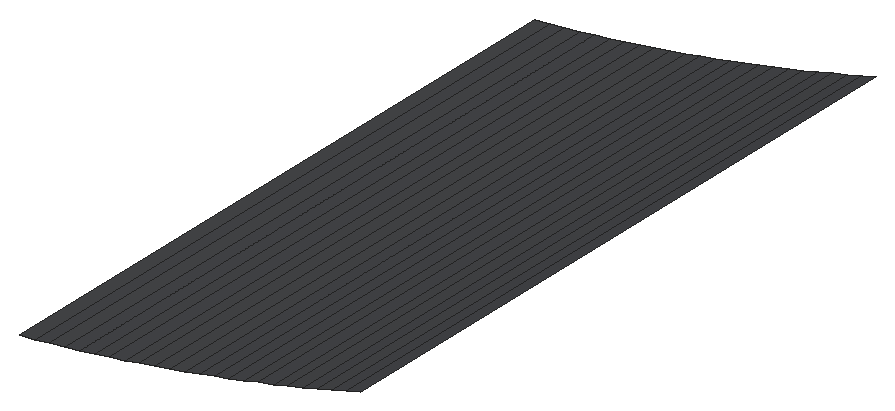
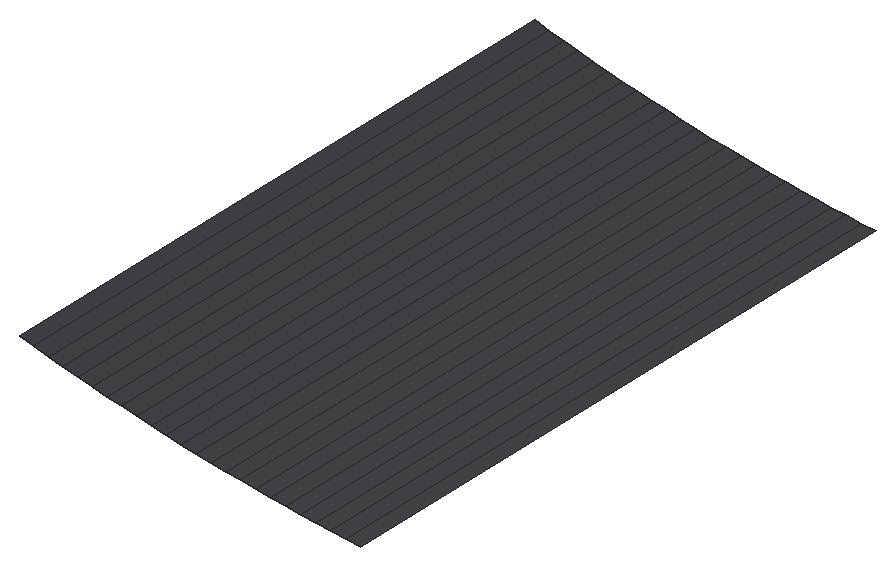
# SketchUp Ruby script. Lengths in inches.
U = 1.inch
M = Sketchup.active_model
def pt(a) = Geom::Point3d.new(a.map { |v| v * U })
def face(e, loops, mat)
  f = e.add_face(loops[0].map { |a| pt(a) })
  loops[1..].each { |l| e.add_face(l.map { |a| pt(a) }).erase! }
  f.material = f.back_material = mat if mat
  f
end
# faces: each face lists its corners as indices into pts; further lists are holes
def faces(e, pts, list, mat = nil) = list.each { |f| face(e, (f[0].is_a?(Array) ? f : [f]).map { |l| l.map { |i| pts[i] } }, mat) }
# xy, xz, yz: faces in a plane at the given z, y or x. An outline is a flat list of corners, or four numbers for a rectangle; further outlines are holes
def ring(l) = l.size == 4 ? [[l[0], l[1]], [l[2], l[1]], [l[2], l[3]], [l[0], l[3]]] : l.each_slice(2).to_a
def flat(e, list, mat, &to3) = list.each { |f| face(e, (f[0].is_a?(Array) ? f : [f]).map { |l| ring(l).map { |u, v| to3.(u, v) } }, mat) }
def xy(e, z, list, mat = nil) = flat(e, list, mat) { |x, y| [x, y, z] }
def xz(e, y, list, mat = nil) = flat(e, list, mat) { |x, z| [x, y, z] }
def yz(e, x, list, mat = nil) = flat(e, list, mat) { |y, z| [x, y, z] }
def lines(e, pts, list) = list.each { |a, b| e.add_line(pt(pts[a]), pt(pts[b])) }
# prism: a flat outline (further loops are holes) pulled along v
def prism(e, loops, v, mat = nil)
  f = face(e, loops, mat); d = Geom::Vector3d.new(v.map { |x| x * U })
  f.pushpull(f.normal.samedirection?(d) ? d.length : -d.length)
end
def box(e, o, s, mat = nil) = prism(e, [[o, [o[0] + s[0], o[1], o[2]], [o[0] + s[0], o[1] + s[1], o[2]], [o[0], o[1] + s[1], o[2]]]], [0, 0, s[2]], mat)
def at(x, y, z, deg = 0) = Geom::Transformation.translation(pt([x, y, z])) * Geom::Transformation.rotation(ORIGIN, Z_AXIS, deg.degrees)
def axes(o, x, y, z) = Geom::Transformation.new([*x, 0, *y, 0, *z, 0, *pt(o).to_a, 1])
def part(name) = M.definitions.add(name)
# library, detail: a bought-in or finely detailed component or shape, given as its bounding box
def library(name, o, s) = part(name).tap { |d| box(d.entities, o, s) }
def detail(e, o, s) = box(e.add_group.entities, o, s)
def put(e, d, t, mat = nil) = e.add_instance(d, t).tap { |i| i.material = mat if mat }
def group(e, t, mat = nil) = e.add_group.tap { |g| g.transformation = t; g.material = mat if mat }.entities
root = M.entities
M.materials.add("1432 AP 8245 TAR ROAD").color = [71, 72, 75]
p = [[540.95,107.37,156.01],[541.23,107.37,156.04],[541.23,95.37,156.04],[540.95,95.37,156.01],[541.51,107.37,156.08],[541.51,95.37,156.08],
  [541.79,107.37,156.11],[541.79,95.37,156.11],[542.07,107.37,156.15],[542.07,95.37,156.15],[542.35,107.37,156.19],[542.35,95.37,156.19],
  [542.63,107.37,156.24],[542.63,95.37,156.24],[542.91,107.37,156.28],[542.91,95.37,156.28],[543.1875,107.37,156.33],[543.1875,95.37,156.33],
  [543.47,107.37,156.38],[543.47,95.37,156.38],[543.75,107.37,156.43],[543.75,95.37,156.43],[544.02,107.37,156.48],[544.02,95.37,156.48],
  [544.3,107.37,156.54],[544.3,95.37,156.54],[544.58,107.37,156.6],[544.58,95.37,156.6],[544.85,107.37,156.66],[544.85,95.37,156.66],
  [545.13,107.37,156.72],[545.13,95.37,156.72],[545.4,107.37,156.79],[545.4,95.37,156.79],[545.68,107.37,156.85],[545.68,95.37,156.85],
  [545.95,107.37,156.92],[545.95,95.37,156.92],[546.23,107.37,156.99],[546.23,95.37,156.99],[546.5,107.37,157.07],[546.5,95.37,157.07],
  [546.77,107.37,157.14],[546.77,95.37,157.14],[547.04,107.37,157.22],[547.04,95.37,157.22],[547.31,107.37,157.3],[547.31,95.37,157.3]]
faces(root,p,[[0,1,2,3],[1,4,5,2],[4,6,7,5],[6,8,9,7],[8,10,11,9],[10,12,13,11],[12,14,15,13],[14,16,17,15],
  [16,18,19,17],[18,20,21,19],[20,22,23,21],[22,24,25,23],[24,26,27,25],[26,28,29,27],[28,30,31,29],[30,32,33,31],
  [32,34,35,33],[34,36,37,35],[36,38,39,37],[38,40,41,39],[40,42,43,41],[42,44,45,43],[44,46,47,45]],"1432 AP 8245 TAR ROAD")
